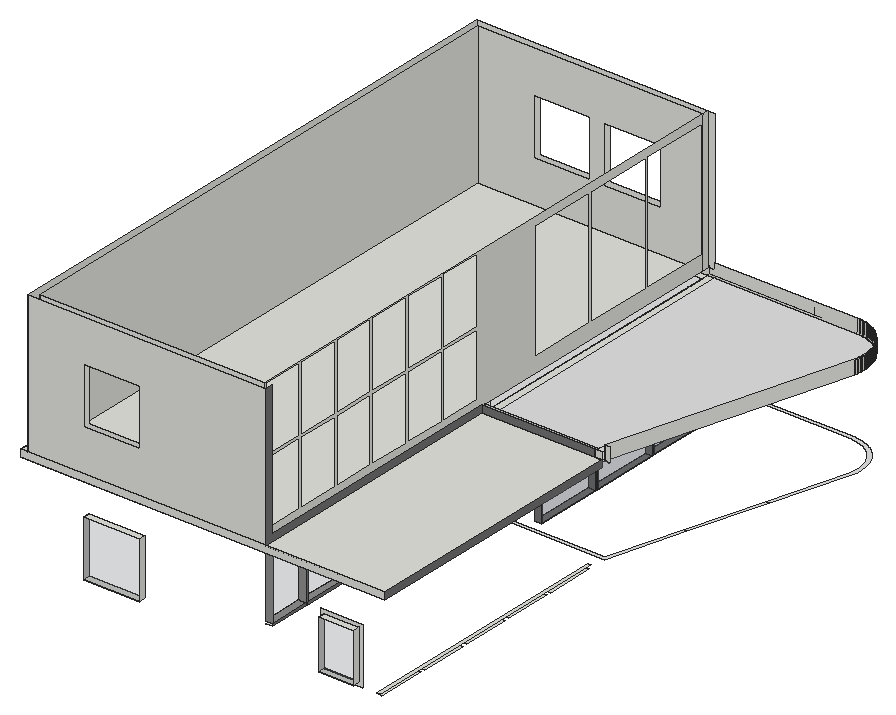
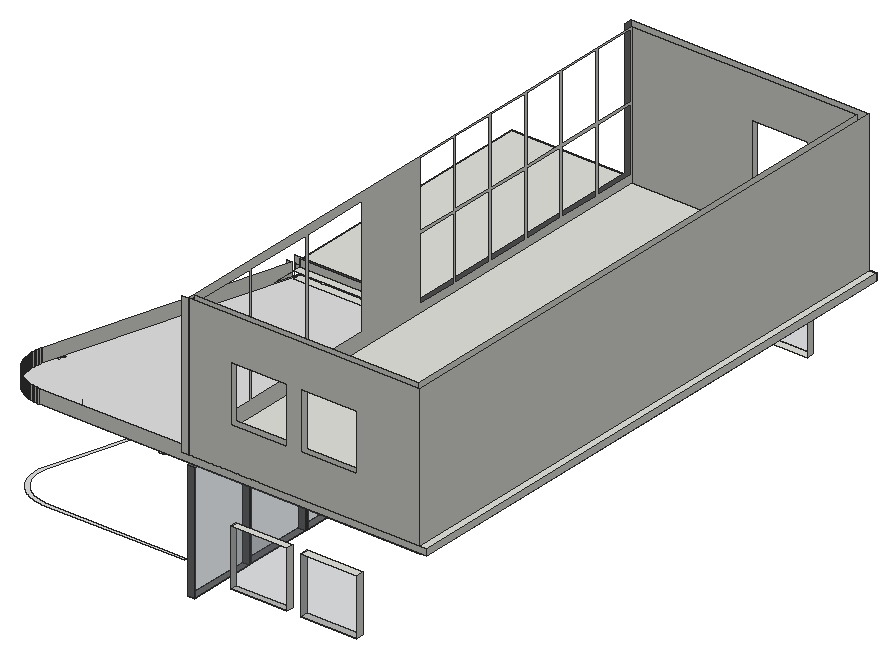
# SketchUp Ruby script. Lengths in inches.
U = 1.inch
M = Sketchup.active_model
def pt(a) = Geom::Point3d.new(a.map { |v| v * U })
def face(e, loops, mat)
  f = e.add_face(loops[0].map { |a| pt(a) })
  loops[1..].each { |l| e.add_face(l.map { |a| pt(a) }).erase! }
  f.material = f.back_material = mat if mat
  f
end
# faces: each face lists its corners as indices into pts; further lists are holes
def faces(e, pts, list, mat = nil) = list.each { |f| face(e, (f[0].is_a?(Array) ? f : [f]).map { |l| l.map { |i| pts[i] } }, mat) }
# xy, xz, yz: faces in a plane at the given z, y or x. An outline is a flat list of corners, or four numbers for a rectangle; further outlines are holes
def ring(l) = l.size == 4 ? [[l[0], l[1]], [l[2], l[1]], [l[2], l[3]], [l[0], l[3]]] : l.each_slice(2).to_a
def flat(e, list, mat, &to3) = list.each { |f| face(e, (f[0].is_a?(Array) ? f : [f]).map { |l| ring(l).map { |u, v| to3.(u, v) } }, mat) }
def xy(e, z, list, mat = nil) = flat(e, list, mat) { |x, y| [x, y, z] }
def xz(e, y, list, mat = nil) = flat(e, list, mat) { |x, z| [x, y, z] }
def yz(e, x, list, mat = nil) = flat(e, list, mat) { |y, z| [x, y, z] }
def lines(e, pts, list) = list.each { |a, b| e.add_line(pt(pts[a]), pt(pts[b])) }
# prism: a flat outline (further loops are holes) pulled along v
def prism(e, loops, v, mat = nil)
  f = face(e, loops, mat); d = Geom::Vector3d.new(v.map { |x| x * U })
  f.pushpull(f.normal.samedirection?(d) ? d.length : -d.length)
end
def box(e, o, s, mat = nil) = prism(e, [[o, [o[0] + s[0], o[1], o[2]], [o[0] + s[0], o[1] + s[1], o[2]], [o[0], o[1] + s[1], o[2]]]], [0, 0, s[2]], mat)
def at(x, y, z, deg = 0) = Geom::Transformation.translation(pt([x, y, z])) * Geom::Transformation.rotation(ORIGIN, Z_AXIS, deg.degrees)
def axes(o, x, y, z) = Geom::Transformation.new([*x, 0, *y, 0, *z, 0, *pt(o).to_a, 1])
def part(name) = M.definitions.add(name)
# library, detail: a bought-in or finely detailed component or shape, given as its bounding box
def library(name, o, s) = part(name).tap { |d| box(d.entities, o, s) }
def detail(e, o, s) = box(e.add_group.entities, o, s)
def put(e, d, t, mat = nil) = e.add_instance(d, t).tap { |i| i.material = mat if mat }
def group(e, t, mat = nil) = e.add_group.tap { |g| g.transformation = t; g.material = mat if mat }.entities
root = M.entities
M.materials.add("Glass_Basic_01").color = [105, 113, 122]
M.materials["Glass_Basic_01"].alpha = 0.25
M.materials.add("M01_Silver_Fog").color = [224, 224, 224]
M.materials.add("M04_Stone_Frost").color = [142, 142, 142]
M.materials.add("M06_Steel_Smoke").color = [114, 114, 114]
xy(root,529,[[204,295,210,353],[204,355,210,413],[204,415,210,473]],"M06_Steel_Smoke")
xy(root,552,[[60,474,108,480],[120,474,168,480]])
xy(root,556,[[300,8,303,49],[300,53,303,94],[300,98,303,139],[300,143,303,184],[300,188,303,229]])
xy(root,558,[[300,6,303,231]])
xy(root,558,[[213,243,305.51,243,324.34,307.35,321.22,307.35,306,255.36,303.26,246,216,246,216,287.79,213,287.79],[321.22,307.35,324.34,307.35,343.2,371.78,340.07,371.78],[340.07,371.78,343.2,371.78,362.06,436.22,362.32,437.22,362.58,438.42,362.79,439.63,362.96,440.85,363.08,442.08,363.16,443.31,363.1875,444.54,363.17,445.77,363.1,447,362.99,448.22,362.83,449.44,362.63,450.66,362.38,451.86,362.08,453.06,361.74,454.24,361.35,455.41,360.92,456.5625,360.45,457.7,359.93,458.82,359.37,459.91,358.77,460.99,358.13,462.03,358.13,462.04,357.45,463.0625,356.73,464.0625,355.97,465.03,355.18,465.98,355.17,465.98,354.35,466.89,353.49,467.76,352.59,468.61,351.67,469.42,350.71,470.19,349.72,470.93,348.71,471.63,347.67,472.29,346.61,472.91,345.52,473.49,344.41,474.03,343.29,474.52,342.14,474.97,340.98,475.38,339.8,475.75,338.61,476.0625,337.41,476.34,336.2,476.5625,334.99,476.74,333.76,476.88,332.53,476.97,331.5,477,210,477,210,474,331.45,474,332.38,473.97,333.49,473.89,334.6,473.77,335.71,473.6,336.8,473.4,337.89,473.15,338.97,472.86,340.04,472.53,341.09,472.16,342.13,471.75,343.16,471.3,344.16,470.82,345.15,470.29,346.11,469.73,347.05,469.13,347.97,468.5,348.87,467.83,349.74,467.125,350.58,466.39,351.39,465.62,352.17,464.83,352.92,464,353.64,463.14,354.33,462.26,354.98,461.36,355.6,460.43,356.18,459.47,356.73,458.5,357.23,457.5,357.7,456.49,358.13,455.46,358.52,454.41,358.875,453.35,359.18,452.28,359.45,451.2,359.68,450.1,359.87,449,360.01,447.89,360.11,446.78,360.17,445.67,360.1875,444.55,360.16,443.43,360.09,442.32,359.98,441.21,359.83,440.1,359.63,439,359.4,437.91,359.17,437.01]],"M01_Silver_Fog")
xy(root,561,[[54,0,102,6],[255,0,285,6]])
xy(root,577,[[204,7,210,43],[204,45,210,81],[204,83,210,119],[204,121,210,157],[204,159,210,195],
  [204,197,210,233]])
xy(root,579,[[204,7,210,43],[204,45,210,81],[204,83,210,119],[204,121,210,157],[204,159,210,195],
  [204,197,210,233]],"M04_Stone_Frost")
xy(root,600,[[60,474,108,480],[120,474,168,480]])
xy(root,603,[[255,0,285,6]])
xy(root,609,[[54,0,102,6]])
xy(root,629,[[204,295,210,353],[204,355,210,413],[204,415,210,473]],"M06_Steel_Smoke")
xy(root,635,[[204,7,210,43],[204,45,210,81],[204,83,210,119],[204,121,210,157],[204,159,210,195],
  [204,197,210,233]])
xy(root,635.24,[[225.03,477.03,225.29,477.03,225.38,477.04,225.46,477.06,225.55,477.08,225.71,477.14,225.87,477.22,225.95,477.27,226.02,477.32,226.08,477.38,226.15,477.4375,226.21,477.5,226.26,477.57,226.32,477.64,226.36,477.72,226.4,477.79,226.44,477.875,226.47,477.96,226.5,478.04,226.54,478.21,226.55,478.3,226.55,478.5625,226.54,478.65,226.52,478.74,226.5,478.82,226.47,478.9,226.4375,478.99,226.4,479.07,226.36,479.14,226.3125,479.22,226.26,479.29,226.2,479.35,226.14,479.42,226.08,479.48,226.01,479.53,225.9375,479.59,225.86,479.63,225.79,479.68,225.71,479.71,225.54,479.77,225.46,479.79,225.37,479.81,225.19,479.83,225.11,479.82,225.02,479.82,224.93,479.81,224.85,479.79,224.76,479.77,224.6,479.71,224.52,479.67,224.4375,479.63,224.36,479.58,224.29,479.53,224.23,479.47,224.16,479.41,224.1,479.35,224.05,479.28,223.99,479.21,223.95,479.13,223.91,479.06,223.87,478.98,223.84,478.9,223.81,478.8125,223.79,478.73,223.77,478.64,223.76,478.55,223.76,478.29,223.77,478.2,223.8125,478.03,223.84,477.95,223.87,477.87,223.95,477.71,224,477.64,224.05,477.56,224.11,477.5,224.17,477.43,224.23,477.37,224.37,477.27,224.45,477.22,224.52,477.18,224.6,477.14,224.68,477.11,224.77,477.08,224.85,477.06,224.94,477.04],[228.34,477.03,228.6,477.03,228.69,477.04,228.78,477.06,228.86,477.08,228.95,477.11,229.03,477.14,229.11,477.18,229.18,477.22,229.26,477.27,229.33,477.32,229.4,477.38,229.46,477.4375,229.52,477.5,229.58,477.57,229.63,477.64,229.67,477.72,229.72,477.79,229.75,477.875,229.79,477.96,229.8125,478.04,229.83,478.125,229.85,478.21,229.87,478.39,229.87,478.47,229.86,478.5625,229.85,478.65,229.83,478.74,229.81,478.82,229.78,478.9,229.75,478.99,229.71,479.07,229.67,479.14,229.62,479.22,229.57,479.29,229.51,479.35,229.45,479.42,229.39,479.48,229.32,479.53,229.25,479.59,229.18,479.63,229.1,479.68,229.02,479.71,228.9375,479.74,228.85,479.77,228.77,479.79,228.68,479.81,228.59,479.82,228.51,479.83,228.42,479.82,228.33,479.82,228.24,479.81,228.16,479.79,228.07,479.77,227.91,479.71,227.75,479.63,227.61,479.53,227.47,479.41,227.41,479.35,227.31,479.21,227.26,479.13,227.22,479.06,227.18,478.98,227.15,478.9,227.12,478.8125,227.1,478.73,227.08,478.64,227.07,478.55,227.07,478.29,227.09,478.2,227.1,478.12,227.125,478.03,227.15,477.95,227.18,477.87,227.26,477.71,227.3125,477.64,227.36,477.56,227.42,477.5,227.48,477.43,227.54,477.37,227.68,477.27,227.76,477.22,227.84,477.18,227.91,477.14,228,477.11,228.08,477.08,228.17,477.06,228.25,477.04]],"M01_Silver_Fog")
xy(root,636,[[0,0,6,231],[6,0,306,0,306,6,210,6,210,231,204,231,204,6,12,6,12,231,6,231],[0,231,6,480],[6,231,6,480,204,480,204,474,12,474,12,231],[204,231,210,231,210,234,306,234,306,240,210,240,210,480,204,480],
  [300,231,306,234]])
xy(root,636,[[12,231,204,474],[210,231,300,234],[[306,234,306,240,210,240,210,480,331.55,480,332.69,479.96,334.03,479.87,335.37,479.72,336.7,479.52,338.02,479.28,339.33,478.98,340.63,478.63,341.92,478.23,343.1875,477.79,344.44,477.29,345.67,476.75,346.88,476.16,348.07,475.53,349.23,474.85,350.37,474.13,351.47,473.37,352.55,472.5625,353.6,471.72,354.61,470.83,355.59,469.91,356.53,468.95,357.39,468,357.4375,467.95,358.3,466.92,359.13,465.86,359.92,464.77,360.66,463.65,360.69,463.59,361.36,462.5,362.02,461.33,362.63,460.13,363.2,458.91,363.71,457.67,364.18,456.41,364.61,455.13,364.98,453.84,365.3,452.53,365.58,451.21,365.8,449.89,365.98,448.55,366.1,447.21,366.17,445.87,366.1875,444.52,366.16,443.18,366.07,441.84,365.94,440.5,365.76,439.16,365.52,437.84,365.24,436.52,364.95,435.42,307.76,240],[358.91,418.8,359,418.81,359.09,418.8125,359.17,418.83,359.26,418.85,359.34,418.87,359.43,418.9,359.51,418.9375,359.58,418.98,359.66,419.02,359.73,419.07,359.87,419.18,359.93,419.24,359.99,419.31,360.09,419.45,360.14,419.53,360.18,419.61,360.21,419.6875,360.24,419.77,360.27,419.85,360.29,419.94,360.3,420.03,360.31,420.11,360.31,420.29,360.3,420.38,360.29,420.46,360.27,420.55,360.24,420.64,360.18,420.8,360.14,420.88,360.09,420.95,360.04,421.03,359.99,421.09,359.93,421.16,359.87,421.22,359.73,421.34,359.66,421.38,359.58,421.43,359.51,421.47,359.43,421.5,359.34,421.53,359.26,421.56,359.17,421.58,359.09,421.59,359,421.6,358.82,421.6,358.73,421.59,358.65,421.58,358.5625,421.56,358.48,421.53,358.39,421.5,358.3125,421.47,358.24,421.43,358.16,421.38,358.09,421.34,357.95,421.22,357.89,421.16,357.83,421.09,357.78,421.03,357.73,420.95,357.68,420.88,357.64,420.8,357.58,420.64,357.55,420.55,357.54,420.46,357.52,420.38,357.51,420.29,357.51,420.11,357.52,420.03,357.54,419.94,357.55,419.85,357.58,419.77,357.61,419.6875,357.64,419.61,357.68,419.53,357.73,419.45,357.83,419.31,357.89,419.24,357.95,419.18,358.09,419.07,358.16,419.02,358.24,418.98,358.3125,418.9375,358.39,418.9,358.48,418.87,358.5625,418.85,358.65,418.83,358.73,418.8125,358.82,418.81],[359.74,421.95,359.92,421.95,360.01,421.96,360.09,421.97,360.18,421.99,360.26,422.02,360.35,422.05,360.43,422.08,360.51,422.12,360.58,422.17,360.65,422.21,360.79,422.33,360.91,422.45,360.96,422.52,361.01,422.6,361.06,422.67,361.1,422.75,361.16,422.91,361.1875,423,361.21,423.08,361.23,423.26,361.23,423.44,361.22,423.52,361.21,423.61,361.1875,423.7,361.16,423.78,361.1,423.94,361.06,424.02,361.01,424.1,360.91,424.24,360.85,424.31,360.79,424.37,360.72,424.43,360.58,424.53,360.51,424.57,360.35,424.65,360.26,424.68,360.18,424.7,360.09,424.72,360.01,424.74,359.92,424.74,359.83,424.75,359.74,424.74,359.66,424.74,359.48,424.7,359.4,424.68,359.32,424.65,359.23,424.61,359.16,424.57,359.08,424.53,359.01,424.48,358.9375,424.43,358.87,424.37,358.81,424.31,358.75,424.24,358.65,424.1,358.6,424.02,358.5625,423.94,358.53,423.86,358.47,423.7,358.46,423.61,358.44,423.52,358.43,423.44,358.43,423.26,358.44,423.17,358.46,423.08,358.47,423,358.5,422.91,358.53,422.83,358.5625,422.75,358.6,422.67,358.65,422.6,358.7,422.52,358.75,422.45,358.87,422.33,358.9375,422.27,359.01,422.21,359.08,422.17,359.16,422.12,359.23,422.08,359.32,422.05,359.48,421.99,359.57,421.97,359.66,421.96]],[358.91,418.8,359,418.81,359.09,418.8125,359.17,418.83,359.26,418.85,359.34,418.87,359.43,418.9,359.51,418.9375,359.58,418.98,359.66,419.02,359.73,419.07,359.87,419.18,359.93,419.24,359.99,419.31,360.09,419.45,360.14,419.53,360.18,419.61,360.21,419.6875,360.24,419.77,360.27,419.85,360.29,419.94,360.3,420.03,360.31,420.11,360.31,420.29,360.3,420.38,360.29,420.46,360.27,420.55,360.24,420.64,360.18,420.8,360.14,420.88,360.09,420.95,360.04,421.03,359.99,421.09,359.93,421.16,359.87,421.22,359.73,421.34,359.66,421.38,359.58,421.43,359.51,421.47,359.43,421.5,359.34,421.53,359.26,421.56,359.17,421.58,359.09,421.59,359,421.6,358.82,421.6,358.73,421.59,358.65,421.58,358.5625,421.56,358.48,421.53,358.39,421.5,358.3125,421.47,358.24,421.43,358.16,421.38,358.09,421.34,357.95,421.22,357.89,421.16,357.83,421.09,357.78,421.03,357.73,420.95,357.68,420.88,357.64,420.8,357.58,420.64,357.55,420.55,357.54,420.46,357.52,420.38,357.51,420.29,357.51,420.11,357.52,420.03,357.54,419.94,357.55,419.85,357.58,419.77,357.61,419.6875,357.64,419.61,357.68,419.53,357.73,419.45,357.83,419.31,357.89,419.24,357.95,419.18,358.09,419.07,358.16,419.02,358.24,418.98,358.3125,418.9375,358.39,418.9,358.48,418.87,358.5625,418.85,358.65,418.83,358.73,418.8125,358.82,418.81],[359.74,421.95,359.92,421.95,360.01,421.96,360.09,421.97,360.18,421.99,360.26,422.02,360.35,422.05,360.43,422.08,360.51,422.12,360.58,422.17,360.65,422.21,360.79,422.33,360.91,422.45,360.96,422.52,361.01,422.6,361.06,422.67,361.1,422.75,361.16,422.91,361.1875,423,361.21,423.08,361.23,423.26,361.23,423.44,361.22,423.52,361.21,423.61,361.1875,423.7,361.16,423.78,361.1,423.94,361.06,424.02,361.01,424.1,360.91,424.24,360.85,424.31,360.79,424.37,360.72,424.43,360.58,424.53,360.51,424.57,360.35,424.65,360.26,424.68,360.18,424.7,360.09,424.72,360.01,424.74,359.92,424.74,359.83,424.75,359.74,424.74,359.66,424.74,359.48,424.7,359.4,424.68,359.32,424.65,359.23,424.61,359.16,424.57,359.08,424.53,359.01,424.48,358.9375,424.43,358.87,424.37,358.81,424.31,358.75,424.24,358.65,424.1,358.6,424.02,358.5625,423.94,358.53,423.86,358.47,423.7,358.46,423.61,358.44,423.52,358.43,423.44,358.43,423.26,358.44,423.17,358.46,423.08,358.47,423,358.5,422.91,358.53,422.83,358.5625,422.75,358.6,422.67,358.65,422.6,358.7,422.52,358.75,422.45,358.87,422.33,358.9375,422.27,359.01,422.21,359.08,422.17,359.16,422.12,359.23,422.08,359.32,422.05,359.48,421.99,359.57,421.97,359.66,421.96]],"M01_Silver_Fog")
xy(root,636,[[306,0,306,6,210,6,210,231,312,231,312,0],[12,6,204,231]],"M06_Steel_Smoke")
xy(root,642,[[0,0,6,480],[210,0,312,231],[12,6,204,474],[210,234,306,240]])
xz(root,0,[[0,636,312,642],[[6,642,210,762],[54,677.98,102,725.98]]])
xz(root,0,[[54,561,102,609],[255,561,285,603]],"Glass_Basic_01")
xz(root,6,[[[252,558,288,606],[255,561,285,603]],[[12,642,204,762],[54,677.98,102,725.98]]])
xz(root,7,[[204,579,210,635]],"M04_Stone_Frost")
xz(root,43,[[204,579,210,635]],"M04_Stone_Frost")
xz(root,45,[[204,579,210,635]],"M04_Stone_Frost")
xz(root,81,[[204,579,210,635]],"M04_Stone_Frost")
xz(root,83,[[204,579,210,635]],"M04_Stone_Frost")
xz(root,119,[[204,579,210,635]],"M04_Stone_Frost")
xz(root,121,[[204,579,210,635]],"M04_Stone_Frost")
xz(root,157,[[204,579,210,635]],"M04_Stone_Frost")
xz(root,159,[[204,579,210,635]],"M04_Stone_Frost")
xz(root,195,[[204,579,210,635]],"M04_Stone_Frost")
xz(root,197,[[204,579,210,635]],"M04_Stone_Frost")
xz(root,231,[[306,636.01,312,642],[306,642,312,648]])
xz(root,231,[[306,636,312,636.01],[210,642,306,648]],"M06_Steel_Smoke")
xz(root,233,[[204,579,210,635]],"M04_Stone_Frost")
xz(root,234,[[210,642,306,648]])
xz(root,240,[[307.76,636,312,636.01],[307.76,636.01,312,648]])
xz(root,295,[[204,529,210,629]],"M06_Steel_Smoke")
xz(root,353,[[204,529,210,629]],"M06_Steel_Smoke")
xz(root,355,[[204,529,210,629]],"M06_Steel_Smoke")
xz(root,413,[[204,529,210,629]],"M06_Steel_Smoke")
xz(root,415,[[204,529,210,629]],"M06_Steel_Smoke")
xz(root,473,[[204,529,210,629]],"M06_Steel_Smoke")
xz(root,474,[[[12,642,204,762],[120,678,168,726],[60,678,108,726]]])
xz(root,480,[[0,636,0,642,210,642,210,648,331.55,648,331.55,636],[[6,642,204,762],[60,678,108,726],[120,678,168,726]],[204,642,210,762]])
xz(root,480,[[60,552,108,600],[120,552,168,600]],"Glass_Basic_01")
yz(root,0,[[0,636,480,642]])
yz(root,6,[[0,642,480,762]])
yz(root,12,[[6,642,474,762]])
yz(root,54,[[0,561,6,609]])
yz(root,60,[[474,552,480,600]])
yz(root,102,[[0,561,6,609]])
yz(root,108,[[474,552,480,600]])
yz(root,120,[[474,552,480,600]])
yz(root,168,[[474,552,480,600]])
yz(root,204,[[[6,642,474,762],[415,655,473,755],[295,655,353,755],[355,655,413,755],[197,705,233,761],[159,705,195,761],[121,705,157,761],[7,705,43,761],[83,705,119,761],[45,705,81,761],[121,649,157,703],[159,649,195,703],[197,649,233,703],[7,649,43,703],[83,649,119,703],[45,649,81,703]],[474,642,480,762]])
yz(root,204,[[295,529,353,629],[355,529,413,629],[415,529,473,629],[7,579,43,635],[45,579,81,635],
  [83,579,119,635],[121,579,157,635],[159,579,195,635],[197,579,233,635]],"Glass_Basic_01")
yz(root,210,[[286.46,568.46,288,589.54]])
yz(root,210,[[295,529,353,629],[355,529,413,629],[415,529,473,629]],"Glass_Basic_01")
yz(root,210,[[7,577,43,579],[45,577,81,579],[83,577,119,579],[121,577,157,579],[159,577,195,579],
  [197,577,233,579],[44,579,45,579,45,635,81,635,81,579,82,579,82,636,44,636],[82,579,83,579,83,635,119,635,119,579,120,579,120,636,82,636],[120,579,121,579,121,635,157,635,157,579,158,579,158,636,120,636],[158,579,159,579,159,635,195,635,195,579,196,579,196,636,158,636],
  [0,642,231,642,231,648,6,648,6,762,0,762]],"M06_Steel_Smoke")
yz(root,255,[[0,561,6,603]])
yz(root,285,[[0,561,6,603]])
yz(root,306,[[231,636,234,636.01],[234,636,240,636.01],[231,636.01,234,648]])
yz(root,312,[[0,636,231,642]],"M06_Steel_Smoke")
p = [[364.95,435.42,648],[307.76,240,648],[307.76,240,636.01],[307.76,240,636],[364.95,435.42,636],[365.24,436.52,648],
  [365.24,436.52,636],[365.52,437.84,648],[365.52,437.84,636],[365.76,439.16,648],[365.76,439.16,636],[365.94,440.5,648],
  [365.94,440.5,636],[366.07,441.84,648],[366.07,441.84,636],[366.16,443.18,648],[366.16,443.18,636],[366.1875,444.52,648],
  [366.1875,444.52,636],[366.17,445.87,648],[366.17,445.87,636],[366.1,447.21,648],[366.1,447.21,636],[365.98,448.55,648],
  [365.98,448.55,636],[365.8,449.89,648],[365.8,449.89,636],[365.58,451.21,648],[365.58,451.21,636],[365.3,452.53,648],
  [365.3,452.53,636],[364.98,453.84,648],[364.98,453.84,636],[364.61,455.13,648],[364.61,455.13,636],[364.18,456.41,648],
  [364.18,456.41,636],[363.71,457.67,648],[363.71,457.67,636],[363.2,458.91,648],[363.2,458.91,636],[362.63,460.13,648],
  [362.63,460.13,636],[362.02,461.33,648],[362.02,461.33,636],[361.36,462.5,648],[361.36,462.5,636],[360.69,463.59,648],
  [360.69,463.59,636],[359.92,464.77,648],[360.66,463.65,648],[360.66,463.65,636],[359.92,464.77,636],[359.13,465.86,648],
  [359.13,465.86,636],[358.3,466.92,648],[358.3,466.92,636],[357.4375,467.95,648],[357.4375,467.95,636],[356.53,468.95,648],
  [357.39,468,648],[357.39,468,636],[356.53,468.95,636],[355.59,469.91,648],[355.59,469.91,636],[354.61,470.83,648],
  [354.61,470.83,636],[353.6,471.72,648],[353.6,471.72,636],[352.55,472.5625,648],[352.55,472.5625,636],[351.47,473.37,648],
  [351.47,473.37,636],[350.37,474.13,648],[350.37,474.13,636],[349.23,474.85,648],[349.23,474.85,636],[348.07,475.53,648],
  [348.07,475.53,636],[346.88,476.16,648],[346.88,476.16,636],[345.67,476.75,648],[345.67,476.75,636],[344.44,477.29,648],
  [344.44,477.29,636],[343.1875,477.79,648],[343.1875,477.79,636],[341.92,478.23,648],[341.92,478.23,636],[340.63,478.63,648],
  [340.63,478.63,636],[339.33,478.98,648],[339.33,478.98,636],[338.02,479.28,648],[338.02,479.28,636],[336.7,479.52,648],
  [336.7,479.52,636],[335.37,479.72,648],[335.37,479.72,636],[334.03,479.87,648],[334.03,479.87,636],[332.69,479.96,648],
  [332.69,479.96,636],[331.55,480,648],[331.55,480,636],[306,260.5,642],[306,240,642],[210,240,642],
  [210,474,642],[210,474,648],[300,474,642],[300,474,648],[306,474,642],[300,240,642],
  [306,240,636.01],[210,240,648]]
faces(root,p,[[0,1,2,3,4],[5,0,4,6],[7,5,6,8],[9,7,8,10],[11,9,10,12],[13,11,12,14],[15,13,14,16],[17,15,16,18],
  [19,17,18,20],[21,19,20,22],[23,21,22,24],[25,23,24,26],[27,25,26,28],[29,27,28,30],[31,29,30,32],[33,31,32,34],
  [35,33,34,36],[37,35,36,38],[39,37,38,40],[41,39,40,42],[43,41,42,44],[45,43,44,46],[47,45,46,48],[49,50,51,52],
  [50,47,48,51],[53,49,52,54],[55,53,54,56],[57,55,56,58],[59,60,61,62],[60,57,58,61],[63,59,62,64],[65,63,64,66],
  [67,65,66,68],[69,67,68,70],[71,69,70,72],[73,71,72,74],[75,73,74,76],[77,75,76,78],[79,77,78,80],[81,79,80,82],
  [83,81,82,84],[85,83,84,86],[87,85,86,88],[89,87,88,90],[91,89,90,92],[93,91,92,94],[95,93,94,96],[97,95,96,98],
  [99,97,98,100],[101,99,100,102],[103,101,102,104]])
lines(root,p,[[105,106],[107,108],[108,109],[110,111],[110,108],[110,112],[113,105],[114,106],[107,115]])
